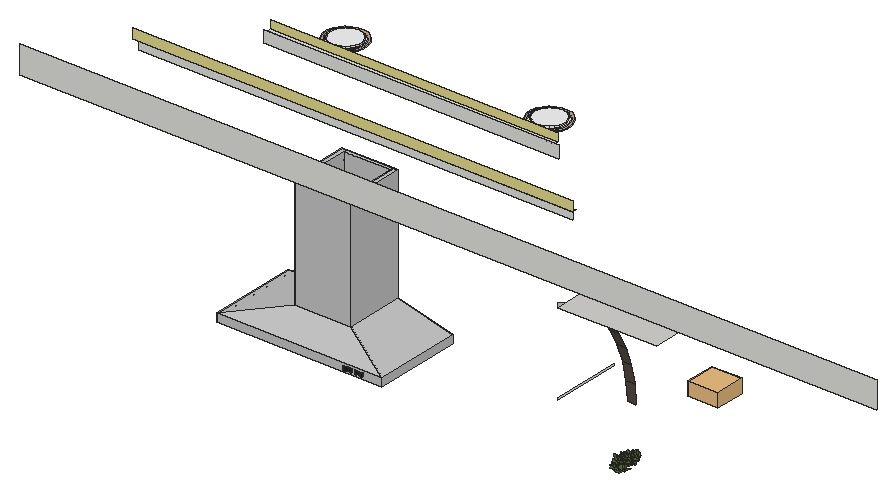
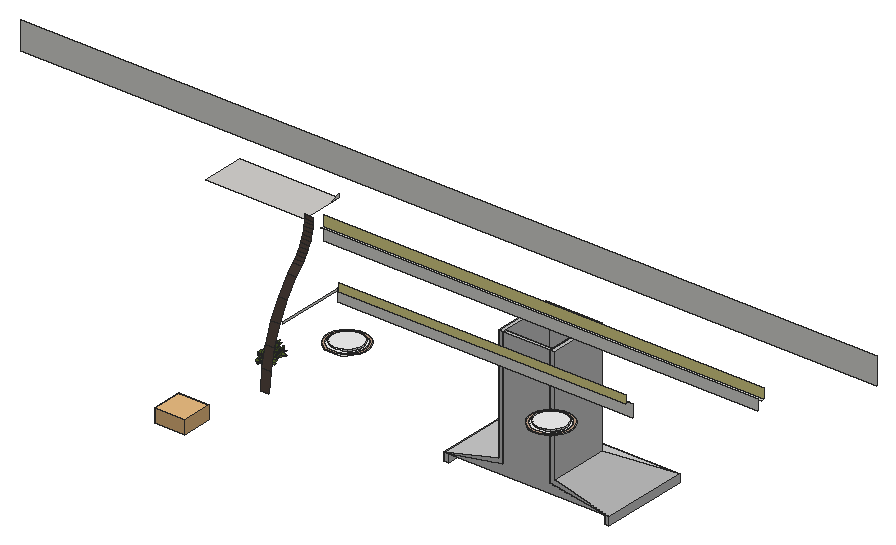
# SketchUp Ruby script. Lengths in inches.
U = 1.inch
M = Sketchup.active_model
def pt(a) = Geom::Point3d.new(a.map { |v| v * U })
def face(e, loops, mat)
  f = e.add_face(loops[0].map { |a| pt(a) })
  loops[1..].each { |l| e.add_face(l.map { |a| pt(a) }).erase! }
  f.material = f.back_material = mat if mat
  f
end
# faces: each face lists its corners as indices into pts; further lists are holes
def faces(e, pts, list, mat = nil) = list.each { |f| face(e, (f[0].is_a?(Array) ? f : [f]).map { |l| l.map { |i| pts[i] } }, mat) }
# xy, xz, yz: faces in a plane at the given z, y or x. An outline is a flat list of corners, or four numbers for a rectangle; further outlines are holes
def ring(l) = l.size == 4 ? [[l[0], l[1]], [l[2], l[1]], [l[2], l[3]], [l[0], l[3]]] : l.each_slice(2).to_a
def flat(e, list, mat, &to3) = list.each { |f| face(e, (f[0].is_a?(Array) ? f : [f]).map { |l| ring(l).map { |u, v| to3.(u, v) } }, mat) }
def xy(e, z, list, mat = nil) = flat(e, list, mat) { |x, y| [x, y, z] }
def xz(e, y, list, mat = nil) = flat(e, list, mat) { |x, z| [x, y, z] }
def yz(e, x, list, mat = nil) = flat(e, list, mat) { |y, z| [x, y, z] }
def lines(e, pts, list) = list.each { |a, b| e.add_line(pt(pts[a]), pt(pts[b])) }
# prism: a flat outline (further loops are holes) pulled along v
def prism(e, loops, v, mat = nil)
  f = face(e, loops, mat); d = Geom::Vector3d.new(v.map { |x| x * U })
  f.pushpull(f.normal.samedirection?(d) ? d.length : -d.length)
end
def box(e, o, s, mat = nil) = prism(e, [[o, [o[0] + s[0], o[1], o[2]], [o[0] + s[0], o[1] + s[1], o[2]], [o[0], o[1] + s[1], o[2]]]], [0, 0, s[2]], mat)
def at(x, y, z, deg = 0) = Geom::Transformation.translation(pt([x, y, z])) * Geom::Transformation.rotation(ORIGIN, Z_AXIS, deg.degrees)
def axes(o, x, y, z) = Geom::Transformation.new([*x, 0, *y, 0, *z, 0, *pt(o).to_a, 1])
def part(name) = M.definitions.add(name)
# library, detail: a bought-in or finely detailed component or shape, given as its bounding box
def library(name, o, s) = part(name).tap { |d| box(d.entities, o, s) }
def detail(e, o, s) = box(e.add_group.entities, o, s)
def put(e, d, t, mat = nil) = e.add_instance(d, t).tap { |i| i.material = mat if mat }
def group(e, t, mat = nil) = e.add_group.tap { |g| g.transformation = t; g.material = mat if mat }.entities
root = M.entities
M.materials.add("2").color = [91, 76, 69]
M.materials.add("Emissive").color = [229, 220, 142]
M.materials.add("Emissive\#1").color = [244, 244, 244]
M.materials.add("[0008_LavenderBlush]").color = [212, 210, 207]
M.materials.add("[Asphalt_New]").color = [85, 106, 44]
M.materials.add("[Blinds_Vertical_Stripe_Gray]").color = [160, 160, 160]
M.materials.add("[Color A01]2").color = [191, 160, 139]
M.materials.add("[Color_002]").color = [198, 198, 198]
M.materials.add("[Color_008]").color = [30, 30, 30]
M.materials.add("white").color = [255, 255, 255]
c1 = part("Component\#59")
xy(c1.entities,0,[[5.79,0,4.75,0.06,3.73,0.22,2.73,0.5,1.77,0.88,0.86,1.37,0,1.95,0.83,2.59,1.74,3.13,2.7,3.56,3.7,3.87,4.74,4.05,5.79,4.12,6.84,4.05,7.87,3.87,8.88,3.56,9.84,3.13,10.74,2.59,11.57,1.95,10.72,1.37,9.8,0.88,8.84,0.5,7.84,0.22,6.82,0.06]],"[Asphalt_New]")
c2 = part("Leaf cluster")
put(c2.entities,c1,axes([10.37,9.23,1.73],[-0.67725,-0.67301,0.29729],[0.61625,-0.73963,-0.27052],[0.40195,0,0.91566]),"[Asphalt_New]")
put(c2.entities,c1,at(0,5.84,1.2),"[Asphalt_New]")
put(c2.entities,c1,axes([11.625,9.72,1.52],[-0.61694,-0.11161,0.77906],[-0.02647,-0.98639,-0.16227],[0.78657,-0.12073,0.60559]),"[Asphalt_New]")
put(c2.entities,c1,axes([13.35,8.05,1.98],[-0.1211,0.99122,-0.05316],[-0.90762,-0.13226,-0.39842],[-0.40195,0,0.91566]),"[Asphalt_New]")
c3 = part("Buttons")
xy(c3.entities,0,[[0,0,0.875,0.75],[0.875,0,1.75,0.75],[2.5,0,3.375,0.75],[3.375,0,4.25,0.75]],"[Color_008]")
xz(c3.entities,0,[[0,0,0,0.25,0.25,0.5,0.875,0],[0.875,0,1.75,0.125,1.75,0],[2.5,0,2.5,0.125,3.375,0],[3.375,0,4,0.5,4.25,0.25,4.25,0]],"[Color_008]")
xz(c3.entities,0.75,[[0,0,0.875,0,0.25,0.5,0,0.25],[0.875,0,1.75,0,1.75,0.125],[2.5,0,3.375,0,2.5,0.125],[3.375,0,4.25,0,4.25,0.25,4,0.5]],"[Color_008]")
yz(c3.entities,0,[[0,0,0.75,0.25]],"[Color_008]")
yz(c3.entities,1.75,[[0,0,0.75,0.125]],"[Color_008]")
yz(c3.entities,2.5,[[0,0,0.75,0.125]],"[Color_008]")
yz(c3.entities,4.25,[[0,0,0.75,0.25]],"[Color_008]")
p = [[0.875,0.75,0],[0.875,0,0],[0.25,0,0.5],[0.25,0.75,0.5],[1.75,0,0.125],[1.75,0.75,0.125],
  [3.375,0,0],[2.5,0,0.125],[2.5,0.75,0.125],[3.375,0.75,0],[4,0.75,0.5],[4,0,0.5],
  [0,0,0.25],[0,0.75,0.25],[4.25,0,0.25],[4.25,0.75,0.25]]
faces(c3.entities,p,[[0,1,2,3],[4,1,0,5],[6,7,8,9],[6,9,10,11],[2,12,13,3],[14,11,10,15]],"[Color_008]")
c4 = part("Range Hood")
xy(c4.entities,0,[[0,0.5,0,24.5,1,24.5,1,1.5,35.25,1.5,35.25,24.5,36.25,24.5,36.25,0.5]],"[Color_002]")
xy(c4.entities,1.75,[[0,0.5,36.25,0.5,36.25,24.5,35.25,24.5,35.25,1.5,1,1.5,1,24.5,0,24.5],[1,23.5,35.25,24.5]],"[Color_002]")
xy(c4.entities,3.93,[[12.97,9.04,23.28,23.5]],"[Blinds_Vertical_Stripe_Gray]")
xy(c4.entities,30,[[11.98,8.42,24.27,8.42,24.27,24.5,23.28,24.5,23.28,9.04,12.97,9.04,12.97,24.5,11.98,24.5],[12.97,23.5,23.28,24.5]],"[Color_002]")
xz(c4.entities,0.5,[[0,0,36.25,1.75]],"[Color_002]")
xz(c4.entities,1.5,[[1,0,35.25,1.75]],"[Color_002]")
xz(c4.entities,8.42,[[11.98,4.75,24.27,30]],"[Color_002]")
xz(c4.entities,9.04,[[12.97,3.93,23.28,30]],"[Color_002]")
xz(c4.entities,23.5,[[1,1.75,35.25,1.75,23.28,3.93,12.97,3.93],[12.97,3.93,23.28,30]],"[Color_002]")
xz(c4.entities,24.5,[[0,0,1,1.75],[35.25,0,36.25,1.75],[0,1.75,11.98,4.75,11.98,30,12.97,30,12.97,3.93,1,1.75],[1,1.75,12.97,3.93,12.97,30,23.28,30,23.28,3.93,35.25,1.75],[35.25,1.75,23.28,3.93,23.28,30,24.27,30,24.27,4.75,36.25,1.75]],"[Color_002]")
yz(c4.entities,0,[[0.5,0,24.5,1.75]],"[Color_002]")
yz(c4.entities,1,[[1.5,0,24.5,1.75]],"[Color_002]")
yz(c4.entities,11.98,[[8.42,4.75,24.5,30]],"[Color_002]")
yz(c4.entities,12.97,[[9.04,3.93,23.5,30],[23.5,3.93,24.5,30]],"[Color_002]")
yz(c4.entities,23.28,[[9.04,3.93,23.5,30],[23.5,3.93,24.5,30]],"[Color_002]")
yz(c4.entities,24.27,[[8.42,4.75,24.5,30]],"[Color_002]")
yz(c4.entities,35.25,[[1.5,0,24.5,1.75]],"[Color_002]")
yz(c4.entities,36.25,[[0.5,0,24.5,1.75]],"[Color_002]")
p = [[0,0.5,1.75],[36.25,0.5,1.75],[24.27,8.42,4.75],[11.98,8.42,4.75],[11.98,24.5,4.75],[0,24.5,1.75],
  [36.25,24.5,1.75],[24.27,24.5,4.75],[35.25,1.5,1.75],[23.28,9.04,3.93],[12.97,9.04,3.93],[11.98,8.42,3.75],
  [1,1.5,1.75],[12.97,23.5,3.93],[1,23.5,1.75],[35.25,23.5,1.75],[23.28,23.5,3.93],[12.97,24.5,3.93],
  [1,24.5,1.75],[35.25,24.5,1.75],[23.28,24.5,3.93]]
faces(c4.entities,p,[[0,1,2,3],[0,3,4,5],[2,1,6,7],[8,9,10,11,12],[12,11,10,13,14],[8,15,16,9],[17,18,14,13],[19,20,16,15]],"[Color_002]")
lines(c4.entities,p,[[3,11]])
put(c4.entities,c3,axes([27.875,0.5,0.5],[1,0,0],[0,0,1],[0,-1,0]))
c5 = part("Range Hood\#1")
put(c5.entities,c4,at(0,-0.5,0))
c6 = library("Group\#200",[0,0,0],[4.97,5,2.25])
xy(root,121.625,[[127.1875,9,148.875,18.35]],"[0008_LavenderBlush]")
xy(root,125.75,[[[44.35,49.27,43.23,49.53,42.22,50.08,41.38,50.86,40.77,51.84,40.4375,52.9375,40.4,54.09,40.66,55.21,41.2,56.22,41.99,57.0625,42.96,57.67,44.0625,58,45.21,58.04,46.33,57.78,47.35,57.24,48.1875,56.45,48.79,55.48,49.13,54.375,49.17,53.23,48.91,52.11,48.36,51.09,47.58,50.25,46.6,49.65,45.5,49.3125],[44.41,49.86,45.4,49.9,46.36,50.19,47.2,50.71,47.88,51.4375,48.35,52.32,48.58,53.28,48.54,54.28,48.26,55.23,47.73,56.08,47,56.76,46.125,57.23,45.16,57.45,44.16,57.42,43.21,57.13,42.36,56.6,41.68,55.88,41.21,55,40.99,54.03,41.02,53.04,41.31,52.08,41.84,51.24,42.5625,50.56,43.44,50.09]],[[89.16,49.27,88.04,49.53,87.03,50.08,86.1875,50.86,85.58,51.84,85.25,52.9375,85.21,54.09,85.47,55.21,86.01,56.22,86.8,57.0625,87.77,57.67,88.875,58,90.02,58.04,91.14,57.78,92.16,57.24,93,56.45,93.6,55.48,93.9375,54.375,93.98,53.23,93.72,52.11,93.17,51.09,92.39,50.25,91.41,49.65,90.3125,49.3125],[89.22,49.86,90.21,49.9,91.17,50.19,92.01,50.71,92.69,51.4375,93.16,52.32,93.39,53.28,93.35,54.28,93.06,55.23,92.54,56.08,91.8125,56.76,90.93,57.23,89.97,57.45,88.97,57.42,88.02,57.13,87.17,56.6,86.49,55.88,86.02,55,85.8,54.03,85.83,53.04,86.12,52.08,86.65,51.24,87.37,50.56,88.25,50.09]]])
xy(root,126,[[[44.41,49.86,43.44,50.09,42.5625,50.56,41.84,51.24,41.31,52.08,41.02,53.04,40.99,54.03,41.21,55,41.68,55.88,42.36,56.6,43.21,57.13,44.16,57.42,45.16,57.45,46.125,57.23,47,56.76,47.73,56.08,48.26,55.23,48.54,54.28,48.58,53.28,48.35,52.32,47.88,51.4375,47.2,50.71,46.36,50.19,45.4,49.9],[44.46,50.34,45.33,50.37,46.16,50.625,46.9,51.08,47.49,51.72,47.9,52.49,48.1,53.33,48.07,54.2,47.82,55.03,47.36,55.77,46.72,56.36,45.96,56.77,45.11,56.97,44.24,56.94,43.41,56.69,42.67,56.23,42.08,55.6,41.67,54.83,41.47,53.98,41.5,53.11,41.75,52.28,42.21,51.54,42.84,50.95,43.61,50.54]],[[89.22,49.86,88.25,50.09,87.37,50.56,86.65,51.24,86.12,52.08,85.83,53.04,85.8,54.03,86.02,55,86.49,55.88,87.17,56.6,88.02,57.13,88.97,57.42,89.97,57.45,90.93,57.23,91.8125,56.76,92.54,56.08,93.06,55.23,93.35,54.28,93.39,53.28,93.16,52.32,92.69,51.4375,92.01,50.71,91.17,50.19,90.21,49.9],[89.27,50.34,90.14,50.37,90.97,50.625,91.71,51.08,92.3,51.72,92.71,52.49,92.91,53.33,92.88,54.2,92.625,55.03,92.17,55.77,91.53,56.36,90.76,56.77,89.92,56.97,89.05,56.94,88.22,56.69,87.48,56.23,86.89,55.6,86.48,54.83,86.28,53.98,86.31,53.11,86.56,52.28,87.02,51.54,87.65,50.95,88.42,50.54]]],"Emissive\#1")
xy(root,126,[[[44.35,49.27,45.5,49.3125,46.6,49.65,47.58,50.25,48.36,51.09,48.91,52.11,49.17,53.23,49.13,54.375,48.79,55.48,48.1875,56.45,47.35,57.24,46.33,57.78,45.21,58.04,44.0625,58,42.96,57.67,41.99,57.0625,41.2,56.22,40.66,55.21,40.4,54.09,40.4375,52.9375,40.77,51.84,41.38,50.86,42.22,50.08,43.23,49.53],[44.41,49.86,43.44,50.09,42.5625,50.56,41.84,51.24,41.31,52.08,41.02,53.04,40.99,54.03,41.21,55,41.68,55.88,42.36,56.6,43.21,57.13,44.16,57.42,45.16,57.45,46.125,57.23,47,56.76,47.73,56.08,48.26,55.23,48.54,54.28,48.58,53.28,48.35,52.32,47.88,51.4375,47.2,50.71,46.36,50.19,45.4,49.9]],[[89.16,49.27,90.3125,49.3125,91.41,49.65,92.39,50.25,93.17,51.09,93.72,52.11,93.98,53.23,93.9375,54.375,93.6,55.48,93,56.45,92.16,57.24,91.14,57.78,90.02,58.04,88.875,58,87.77,57.67,86.8,57.0625,86.01,56.22,85.47,55.21,85.21,54.09,85.25,52.9375,85.58,51.84,86.1875,50.86,87.03,50.08,88.04,49.53],[89.22,49.86,88.25,50.09,87.37,50.56,86.65,51.24,86.12,52.08,85.83,53.04,85.8,54.03,86.02,55,86.49,55.88,87.17,56.6,88.02,57.13,88.97,57.42,89.97,57.45,90.93,57.23,91.8125,56.76,92.54,56.08,93.06,55.23,93.35,54.28,93.39,53.28,93.16,52.32,92.69,51.4375,92.01,50.71,91.17,50.19,90.21,49.9]]],"[Color A01]2")
xy(root,126.375,[[44.46,50.34,43.61,50.54,42.84,50.95,42.21,51.54,41.75,52.28,41.5,53.11,41.47,53.98,41.67,54.83,42.08,55.6,42.67,56.23,43.41,56.69,44.24,56.94,45.11,56.97,45.96,56.77,46.72,56.36,47.36,55.77,47.82,55.03,48.07,54.2,48.1,53.33,47.9,52.49,47.49,51.72,46.9,51.08,46.16,50.625,45.33,50.37],[89.27,50.34,88.42,50.54,87.65,50.95,87.02,51.54,86.56,52.28,86.31,53.11,86.28,53.98,86.48,54.83,86.89,55.6,87.48,56.23,88.22,56.69,89.05,56.94,89.92,56.97,90.76,56.77,91.53,56.36,92.17,55.77,92.625,55.03,92.88,54.2,92.91,53.33,92.71,52.49,92.3,51.72,91.71,51.08,90.97,50.625,90.14,50.37]],"Emissive\#1")
xy(root,128.22,[[18.79,27.67,115.58,28.36]])
xy(root,128.6875,[[35.66,43.66,98.72,44.53]])
xz(root,9,[[9,126,197.1875,132]])
xz(root,27.67,[[18.79,128.22,115.58,130.4375]],"Emissive")
xz(root,28.36,[[19.48,126,114.89,128.22]])
xz(root,43.66,[[34.78,126,99.59,128.6875]])
xz(root,44.53,[[35.66,128.6875,98.72,130.4375]],"Emissive")
yz(root,127.1875,[[9,103.38,24.3,103.78],[9,121.625,10.92,121.625,9,122.4375],[18.35,121.625,18.37,121.625,18.37,121.69,18.35,122.4375]])
p = [[125.3125,30.54,93.04],[125.3125,30.14,97.33],[127.1875,30.14,97.33],[127.1875,30.54,93.04],[125.3125,29.16,101.52],[127.1875,29.16,101.52],
  [125.3125,27.63,105.54],[127.1875,27.63,105.54],[125.3125,25.57,109.32],[127.1875,25.57,109.32],[125.3125,23.03,112.8],[127.1875,23.03,112.8],
  [125.3125,21.54,114.35],[127.1875,21.54,114.35],[127.1875,21.04,114.9],[125.3125,21.04,114.9],[127.1875,20.58,115.48],[125.3125,20.58,115.48],
  [127.1875,20.16,116.09],[125.3125,20.16,116.09],[127.1875,19.77,116.73],[125.3125,19.77,116.73],[127.1875,19.4375,117.39],[125.3125,19.4375,117.39],
  [127.1875,19.14,118.08],[125.3125,19.14,118.08],[127.1875,18.89,118.78],[125.3125,18.89,118.78],[127.1875,18.6875,119.49],[125.3125,18.6875,119.49],
  [127.1875,18.53,120.22],[125.3125,18.53,120.22],[127.1875,18.43,120.95],[125.3125,18.43,120.95],[127.1875,18.37,121.625],[125.3125,18.37,121.69],
  [127.1875,18.37,121.69],[127.1875,18.35,122.4375],[125.3125,18.35,122.4375],[44.35,49.27,126],[43.23,49.53,126],[43.23,49.53,125.75],
  [44.35,49.27,125.75],[45.5,49.3125,126],[45.5,49.3125,125.75],[46.6,49.65,126],[46.6,49.65,125.75],[89.16,49.27,126],
  [88.04,49.53,126],[88.04,49.53,125.75],[89.16,49.27,125.75],[90.3125,49.3125,126],[90.3125,49.3125,125.75],[91.41,49.65,126],
  [91.41,49.65,125.75],[42.22,50.08,126],[42.22,50.08,125.75],[87.03,50.08,126],[87.03,50.08,125.75],[47.58,50.25,126],
  [47.58,50.25,125.75],[92.39,50.25,126],[92.39,50.25,125.75],[43.44,50.09,126],[44.41,49.86,126],[44.41,49.86,125.75],
  [43.44,50.09,125.75],[45.4,49.9,126],[45.4,49.9,125.75],[46.36,50.19,126],[46.36,50.19,125.75],[88.25,50.09,126],
  [89.22,49.86,126],[89.22,49.86,125.75],[88.25,50.09,125.75],[90.21,49.9,126],[90.21,49.9,125.75],[91.17,50.19,126],
  [91.17,50.19,125.75],[41.38,50.86,126],[41.38,50.86,125.75],[42.5625,50.56,126],[42.5625,50.56,125.75],[86.1875,50.86,126],
  [86.1875,50.86,125.75],[87.37,50.56,126],[87.37,50.56,125.75],[47.2,50.71,126],[47.2,50.71,125.75],[92.01,50.71,126],
  [92.01,50.71,125.75],[48.36,51.09,126],[48.36,51.09,125.75],[93.17,51.09,126],[93.17,51.09,125.75],[41.84,51.24,126],
  [41.84,51.24,125.75],[86.65,51.24,126],[86.65,51.24,125.75],[47.88,51.4375,126],[47.88,51.4375,125.75],[92.69,51.4375,126],
  [92.69,51.4375,125.75],[40.77,51.84,126],[40.77,51.84,125.75],[85.58,51.84,126],[85.58,51.84,125.75],[48.91,52.11,126],
  [48.91,52.11,125.75],[93.72,52.11,126],[93.72,52.11,125.75],[41.31,52.08,126],[41.31,52.08,125.75],[86.12,52.08,126],
  [86.12,52.08,125.75],[48.35,52.32,126],[48.35,52.32,125.75],[93.16,52.32,126],[93.16,52.32,125.75],[40.4375,52.9375,126],
  [40.4375,52.9375,125.75],[85.25,52.9375,126],[85.25,52.9375,125.75],[41.02,53.04,126],[41.02,53.04,125.75],[49.17,53.23,126],
  [49.17,53.23,125.75],[85.83,53.04,126],[85.83,53.04,125.75],[93.98,53.23,126],[93.98,53.23,125.75],[48.58,53.28,126],
  [48.58,53.28,125.75],[93.39,53.28,126],[93.39,53.28,125.75],[40.4,54.09,126],[40.4,54.09,125.75],[85.21,54.09,126],
  [85.21,54.09,125.75],[40.99,54.03,126],[40.99,54.03,125.75],[85.8,54.03,126],[85.8,54.03,125.75],[49.13,54.375,126],
  [49.13,54.375,125.75],[93.9375,54.375,126],[93.9375,54.375,125.75],[48.54,54.28,126],[48.54,54.28,125.75],[93.35,54.28,126],
  [93.35,54.28,125.75],[41.21,55,126],[41.21,55,125.75],[86.02,55,126],[86.02,55,125.75],[40.66,55.21,126],
  [40.66,55.21,125.75],[85.47,55.21,126],[85.47,55.21,125.75],[48.26,55.23,126],[48.26,55.23,125.75],[93.06,55.23,126],
  [93.06,55.23,125.75],[48.79,55.48,126],[48.79,55.48,125.75],[93.6,55.48,126],[93.6,55.48,125.75],[41.68,55.88,126],
  [41.68,55.88,125.75],[86.49,55.88,126],[86.49,55.88,125.75],[41.2,56.22,126],[41.2,56.22,125.75],[47.73,56.08,126],
  [47.73,56.08,125.75],[86.01,56.22,126],[86.01,56.22,125.75],[92.54,56.08,126],[92.54,56.08,125.75],[48.1875,56.45,126],
  [48.1875,56.45,125.75],[93,56.45,126],[93,56.45,125.75],[42.36,56.6,126],[42.36,56.6,125.75],[87.17,56.6,126],
  [87.17,56.6,125.75],[47,56.76,126],[47,56.76,125.75],[91.8125,56.76,126],[91.8125,56.76,125.75],[44.46,50.34,126],
  [43.61,50.54,126],[43.61,50.54,126.375],[44.46,50.34,126.375],[45.33,50.37,126],[45.33,50.37,126.375],[89.27,50.34,126],
  [88.42,50.54,126],[88.42,50.54,126.375],[89.27,50.34,126.375],[90.14,50.37,126],[90.14,50.37,126.375],[46.16,50.625,126],
  [46.16,50.625,126.375],[90.97,50.625,126],[90.97,50.625,126.375],[42.84,50.95,126],[42.84,50.95,126.375],[87.65,50.95,126],
  [87.65,50.95,126.375],[46.9,51.08,126],[46.9,51.08,126.375],[91.71,51.08,126],[91.71,51.08,126.375],[42.21,51.54,126],
  [42.21,51.54,126.375],[87.02,51.54,126],[87.02,51.54,126.375],[47.49,51.72,126],[47.49,51.72,126.375],[92.3,51.72,126],
  [92.3,51.72,126.375],[41.75,52.28,126],[41.75,52.28,126.375],[86.56,52.28,126],[86.56,52.28,126.375],[47.9,52.49,126],
  [47.9,52.49,126.375],[92.71,52.49,126],[92.71,52.49,126.375],[41.5,53.11,126],[41.5,53.11,126.375],[86.31,53.11,126],
  [86.31,53.11,126.375],[48.1,53.33,126],[48.1,53.33,126.375],[92.91,53.33,126],[92.91,53.33,126.375],[41.47,53.98,126],
  [41.47,53.98,126.375],[86.28,53.98,126],[86.28,53.98,126.375],[48.07,54.2,126],[48.07,54.2,126.375],[92.88,54.2,126],
  [92.88,54.2,126.375],[41.67,54.83,126],[41.67,54.83,126.375],[86.48,54.83,126],[86.48,54.83,126.375],[47.82,55.03,126],
  [47.82,55.03,126.375],[92.625,55.03,126],[92.625,55.03,126.375],[42.08,55.6,126],[42.08,55.6,126.375],[86.89,55.6,126],
  [86.89,55.6,126.375],[47.36,55.77,126],[47.36,55.77,126.375],[92.17,55.77,126],[92.17,55.77,126.375],[42.67,56.23,126],
  [42.67,56.23,126.375],[87.48,56.23,126],[87.48,56.23,126.375],[46.72,56.36,126],[46.72,56.36,126.375],[91.53,56.36,126],
  [91.53,56.36,126.375],[43.41,56.69,126],[43.41,56.69,126.375],[88.22,56.69,126],[88.22,56.69,126.375],[125.3125,20.04,115.9],
  [127.1875,20.04,115.9]]
faces(root,p,[[0,1,2,3],[1,4,5,2],[4,6,7,5],[6,8,9,7],[8,10,11,9],[10,12,13,11],[14,13,12,15],[16,14,15,17],
  [18,16,17,19],[20,18,19,21],[22,20,21,23],[24,22,23,25],[26,24,25,27],[28,26,27,29],[30,28,29,31],[32,30,31,33],
  [34,32,33,35,36],[37,36,35,38]],"2")
faces(root,p,[[39,40,41,42],[43,39,42,44],[45,43,44,46],[47,48,49,50],[51,47,50,52],[53,51,52,54],[40,55,56,41],[48,57,58,49],
  [59,45,46,60],[61,53,54,62],[63,64,65,66],[64,67,68,65],[67,69,70,68],[71,72,73,74],[72,75,76,73],[75,77,78,76],
  [55,79,80,56],[81,63,66,82],[57,83,84,58],[85,71,74,86],[69,87,88,70],[77,89,90,78],[91,59,60,92],[93,61,62,94],
  [95,81,82,96],[97,85,86,98],[87,99,100,88],[89,101,102,90],[79,103,104,80],[83,105,106,84],[107,91,92,108],[109,93,94,110],
  [111,95,96,112],[113,97,98,114],[99,115,116,100],[101,117,118,102],[103,119,120,104],[105,121,122,106],[123,111,112,124],[125,107,108,126],
  [127,113,114,128],[129,109,110,130],[115,131,132,116],[117,133,134,118],[119,135,136,120],[121,137,138,122],[139,123,124,140],[141,127,128,142],
  [143,125,126,144],[145,129,130,146],[131,147,148,132],[133,149,150,134],[151,139,140,152],[153,141,142,154],[135,155,156,136],[137,157,158,138],
  [147,159,160,148],[149,161,162,150],[163,143,144,164],[165,145,146,166],[167,151,152,168],[169,153,154,170],[155,171,172,156],[159,173,174,160],
  [157,175,176,158],[161,177,178,162],[179,163,164,180],[181,165,166,182],[183,167,168,184],[185,169,170,186],[173,187,188,174],[177,189,190,178]])
faces(root,p,[[191,192,193,194],[195,191,194,196],[197,198,199,200],[201,197,200,202],[203,195,196,204],[205,201,202,206],[192,207,208,193],[198,209,210,199],
  [211,203,204,212],[213,205,206,214],[207,215,216,208],[209,217,218,210],[219,211,212,220],[221,213,214,222],[215,223,224,216],[217,225,226,218],
  [227,219,220,228],[229,221,222,230],[223,231,232,224],[225,233,234,226],[235,227,228,236],[237,229,230,238],[231,239,240,232],[233,241,242,234],
  [243,235,236,244],[245,237,238,246],[239,247,248,240],[241,249,250,242],[251,243,244,252],[253,245,246,254],[247,255,256,248],[249,257,258,250],
  [259,251,252,260],[261,253,254,262],[255,263,264,256],[257,265,266,258],[267,259,260,268],[269,261,262,270],[263,271,272,264],[265,273,274,266]],"Emissive\#1")
lines(root,p,[[275,276]])
put(root,c1,axes([137.23,14.35,90.7],[-0.15155,-0.00971,-0.00946],[0.01213,-0.13895,-0.07089],[-0.00352,-0.06102,0.16292]),"[Asphalt_New]")
put(root,c2,axes([138.14,14.47,90.66],[-0.10136,0.11337,0],[-0.11337,-0.10136,0],[0,0,0.17792]),"white")
put(root,c1,axes([136.85,15.16,90.88],[-0.12443,-0.07482,0.0529],[0.06418,-0.13158,-0.04813],[0.05936,-0.01458,0.16292]),"[Asphalt_New]")
put(root,c1,axes([135.92,15,90.61],[-0.09292,-0.02137,0.13861],[0.00305,-0.15002,-0.02887],[0.12035,-0.0127,0.10775]),"[Asphalt_New]")
put(root,c1,axes([134.18,14.33,90.56],[0.1519,0.00716,0],[-0.00716,0.1519,0],[0,0,0.17792]),"[Asphalt_New]")
put(root,c2,axes([134.89,14.14,90.52],[0.1271,-0.08349,0],[0.08349,0.1271,0],[0,0,0.17792]),"white")
put(root,c1,axes([137.05,15.1875,90.85],[-0.09516,0.0059,0.13861],[-0.03969,-0.14471,-0.02887],[0.11178,-0.04636,0.10775]),"[Asphalt_New]")
put(root,c1,axes([137.3125,15.38,90.91],[-0.15155,-0.00971,-0.00946],[0.01213,-0.13895,-0.07089],[-0.00352,-0.06102,0.16292]),"[Asphalt_New]")
put(root,c2,axes([135.57,13.375,91.2],[0.12994,0.079,0],[-0.079,0.12994,0],[0,0,0.17792]),"white")
put(root,c1,axes([135.2,15.04,90.79],[0.14768,-0.03627,0],[0.03627,0.14768,0],[0,0,0.17792]),"[Asphalt_New]")
put(root,c1,axes([135.81,16.02,90.87],[-0.09806,-0.10708,0.0529],[0.09891,-0.10794,-0.04813],[0.06106,0.00288,0.16292]),"[Asphalt_New]")
put(root,c2,axes([138.22,15.57,90.87],[-0.10136,0.11337,0],[-0.11337,-0.10136,0],[0,0,0.17792]),"white")
put(root,c1,axes([136.19,16.34,90.65],[-0.09806,-0.10708,0.0529],[0.09891,-0.10794,-0.04813],[0.06106,0.00288,0.16292]),"[Asphalt_New]")
put(root,c2,axes([135.73,17.0625,90.52],[-0.06975,-0.13513,0],[0.13513,-0.06975,0],[0,0,0.17792]),"white")
put(root,c2,axes([135.96,13.875,91.2],[0.12994,0.079,0],[-0.079,0.12994,0],[0,0,0.17792]),"white")
put(root,c1,axes([136.1875,14.76,90.7],[-0.0255,0.1497,-0.00946],[-0.13692,-0.02659,-0.07089],[-0.06106,-0.00288,0.16292]),"[Asphalt_New]")
put(root,c1,axes([135.99,16.11,90.83],[-0.09292,-0.02137,0.13861],[0.00305,-0.15002,-0.02887],[0.12035,-0.0127,0.10775]),"[Asphalt_New]")
put(root,c1,axes([134.26,15.43,90.77],[0.1519,0.00716,0],[-0.00716,0.1519,0],[0,0,0.17792]),"[Asphalt_New]")
put(root,c2,axes([137.2,15.98,90.66],[-0.10136,0.11337,0],[-0.11337,-0.10136,0],[0,0,0.17792]),"white")
put(root,c2,axes([136,14.17,91.2],[0.12739,0.08305,0],[-0.08305,0.12739,0],[0,0,0.17792]),"white")
put(root,c1,axes([136.375,16.42,90.61],[-0.09292,-0.02137,0.13861],[0.00305,-0.15002,-0.02887],[0.12035,-0.0127,0.10775]),"[Asphalt_New]")
put(root,c2,axes([136.93,14.44,91.07],[0.07604,0.1317,0],[-0.1317,0.07604,0],[0,0,0.17792]),"white")
put(root,c1,axes([136.5,15.46,91.16],[-0.00408,0.09525,0.13861],[-0.14807,0.02435,-0.02887],[-0.03442,-0.11602,0.10775]),"[Asphalt_New]")
put(root,c1,axes([134.97,16.52,90.61],[-0.09292,-0.02137,0.13861],[0.00305,-0.15002,-0.02887],[0.12035,-0.0127,0.10775]),"[Asphalt_New]")
put(root,c1,axes([134.64,15.75,90.56],[0.1519,0.00716,0],[-0.00716,0.1519,0],[0,0,0.17792]),"[Asphalt_New]")
put(root,c1,axes([135.58,16.07,91],[0.14768,-0.03627,0],[0.03627,0.14768,0],[0,0,0.17792]),"[Asphalt_New]")
put(root,c1,axes([136.45,15.66,91.19],[-0.08742,0.11593,0.0529],[-0.12415,-0.07758,-0.04813],[-0.0083,-0.06056,0.16292]),"[Asphalt_New]")
put(root,c1,axes([136.375,16.875,90.88],[-0.12443,-0.07482,0.0529],[0.06418,-0.13158,-0.04813],[0.05936,-0.01458,0.16292]),"[Asphalt_New]")
put(root,c2,axes([136.37,14.68,91.2],[0.12739,0.08305,0],[-0.08305,0.12739,0],[0,0,0.17792]),"white")
put(root,c1,axes([136.16,17.29,91.1],[-0.02064,-0.15066,0],[0.15066,-0.02064,0],[0,0,0.17792]),"[Asphalt_New]")
put(root,c1,axes([136.58,16.9,90.85],[-0.09516,0.0059,0.13861],[-0.03969,-0.14471,-0.02887],[0.11178,-0.04636,0.10775]),"[Asphalt_New]")
put(root,c1,axes([136.85,16.16,91.19],[-0.08742,0.11593,0.0529],[-0.12415,-0.07758,-0.04813],[-0.0083,-0.06056,0.16292]),"[Asphalt_New]")
put(root,c1,axes([136.27,15.86,90.91],[-0.0255,0.1497,-0.00946],[-0.13692,-0.02659,-0.07089],[-0.06106,-0.00288,0.16292]),"[Asphalt_New]")
put(root,c1,axes([136.37,17.59,90.65],[-0.09806,-0.10708,0.0529],[0.09891,-0.10794,-0.04813],[0.06106,0.00288,0.16292]),"[Asphalt_New]")
put(root,c1,axes([135.25,17.68,90.65],[-0.09806,-0.10708,0.0529],[0.09891,-0.10794,-0.04813],[0.06106,0.00288,0.16292]),"[Asphalt_New]")
put(root,c1,axes([134.72,16.75,90.79],[0.14768,-0.03627,0],[0.03627,0.14768,0],[0,0,0.17792]),"[Asphalt_New]")
put(root,c1,axes([136.86,16.29,91.16],[-0.00707,0.09508,0.13861],[-0.14876,0.01968,-0.02887],[-0.03076,-0.11704,0.10775]),"[Asphalt_New]")
put(root,c1,axes([136.81,16.49,91.19],[-0.09102,0.11312,0.0529],[-0.12166,-0.08144,-0.04813],[-0.00639,-0.06079,0.16292]),"[Asphalt_New]")
put(root,c1,axes([136.65,16.18,90.7],[-0.0255,0.1497,-0.00946],[-0.13692,-0.02659,-0.07089],[-0.06106,-0.00288,0.16292]),"[Asphalt_New]")
put(root,c2,axes([134.79,18.57,90.52],[-0.06975,-0.13513,0],[0.13513,-0.06975,0],[0,0,0.17792]),"white")
put(root,c2,axes([137.66,17.23,90.66],[-0.10136,0.11337,0],[-0.11337,-0.10136,0],[0,0,0.17792]),"white")
put(root,c1,axes([135.25,16.27,90.7],[-0.0255,0.1497,-0.00946],[-0.13692,-0.02659,-0.07089],[-0.06106,-0.00288,0.16292]),"[Asphalt_New]")
put(root,c2,axes([134.66,17.15,91.21],[0.09591,-0.11801,0],[0.11801,0.09591,0],[0,0,0.17792]),"white")
put(root,c1,axes([136.56,17.67,90.61],[-0.09292,-0.02137,0.13861],[0.00305,-0.15002,-0.02887],[0.12035,-0.0127,0.10775]),"[Asphalt_New]")
put(root,c1,axes([135.4375,17.76,90.61],[-0.09292,-0.02137,0.13861],[0.00305,-0.15002,-0.02887],[0.12035,-0.0127,0.10775]),"[Asphalt_New]")
put(root,c1,axes([134.82,17,90.56],[0.1519,0.00716,0],[-0.00716,0.1519,0],[0,0,0.17792]),"[Asphalt_New]")
put(root,c1,axes([135.49,18.24,90.4375],[-0.09806,-0.10708,0.0529],[0.09891,-0.10794,-0.04813],[0.06106,0.00288,0.16292]),"[Asphalt_New]")
put(root,c1,axes([136.52,18.26,90.65],[-0.09806,-0.10708,0.0529],[0.09891,-0.10794,-0.04813],[0.06106,0.00288,0.16292]),"[Asphalt_New]")
put(root,c1,axes([137.18,17,91.19],[-0.09102,0.11312,0.0529],[-0.12166,-0.08144,-0.04813],[-0.00639,-0.06079,0.16292]),"[Asphalt_New]")
put(root,c2,axes([137.9,17.79,90.44],[-0.10136,0.11337,0],[-0.11337,-0.10136,0],[0,0,0.17792]),"white")
put(root,c1,axes([135.68,18.32,90.4],[-0.09292,-0.02137,0.13861],[0.00305,-0.15002,-0.02887],[0.12035,-0.0127,0.10775]),"[Asphalt_New]")
put(root,c1,axes([135.52,17.81,90.79],[0.14768,-0.03627,0],[0.03627,0.14768,0],[0,0,0.17792]),"[Asphalt_New]")
put(root,c1,axes([136.71,18.35,90.61],[-0.09292,-0.02137,0.13861],[0.00305,-0.15002,-0.02887],[0.12035,-0.0127,0.10775]),"[Asphalt_New]")
put(root,c2,axes([135.83,16.25,90.67],[0.12994,0.079,0],[-0.079,0.12994,0],[0,0,0.17792]),"white")
put(root,c1,axes([133.9375,17.65,90.34],[0.1519,0.00716,0],[-0.00716,0.1519,0],[0,0,0.17792]),"[Asphalt_New]")
put(root,c1,axes([134.97,17.67,90.56],[0.1519,0.00716,0],[-0.00716,0.1519,0],[0,0,0.17792]),"[Asphalt_New]")
put(root,c1,axes([136.83,17.43,90.7],[-0.0255,0.1497,-0.00946],[-0.13692,-0.02659,-0.07089],[-0.06106,-0.00288,0.16292]),"[Asphalt_New]")
put(root,c2,axes([135.26,19.82,90.52],[-0.06975,-0.13513,0],[0.13513,-0.06975,0],[0,0,0.17792]),"white")
put(root,c1,axes([135.71,17.52,90.7],[-0.0255,0.1497,-0.00946],[-0.13692,-0.02659,-0.07089],[-0.06106,-0.00288,0.16292]),"[Asphalt_New]")
put(root,c2,axes([136.17,17.06,90.67],[0.12739,0.08305,0],[-0.08305,0.12739,0],[0,0,0.17792]),"white")
put(root,c2,axes([135.5,20.38,90.31],[-0.06975,-0.13513,0],[0.13513,-0.06975,0],[0,0,0.17792]),"white")
put(root,c1,axes([135.95,18.08,90.48],[-0.0255,0.1497,-0.00946],[-0.13692,-0.02659,-0.07089],[-0.06106,-0.00288,0.16292]),"[Asphalt_New]")
put(root,c5,axes([51.9375,9.4,92.13],[1,0,0],[0,0.8084,0],[0,0,1]))
put(root,c1,axes([136.77,18.34,90.63],[-0.00408,0.09525,0.13861],[-0.14807,0.02435,-0.02887],[-0.03442,-0.11602,0.10775]),"[Asphalt_New]")
put(root,c1,axes([136.72,18.54,90.67],[-0.08742,0.11593,0.0529],[-0.12415,-0.07758,-0.04813],[-0.0083,-0.06056,0.16292]),"[Asphalt_New]")
put(root,c1,axes([136.98,19.37,90.67],[-0.09102,0.11312,0.0529],[-0.12166,-0.08144,-0.04813],[-0.00639,-0.06079,0.16292]),"[Asphalt_New]")
put(root,c6,axes([130.04,47.8,90.98],[0,-1.3225,0],[1.3225,0,0],[0,0,1.3225]))
